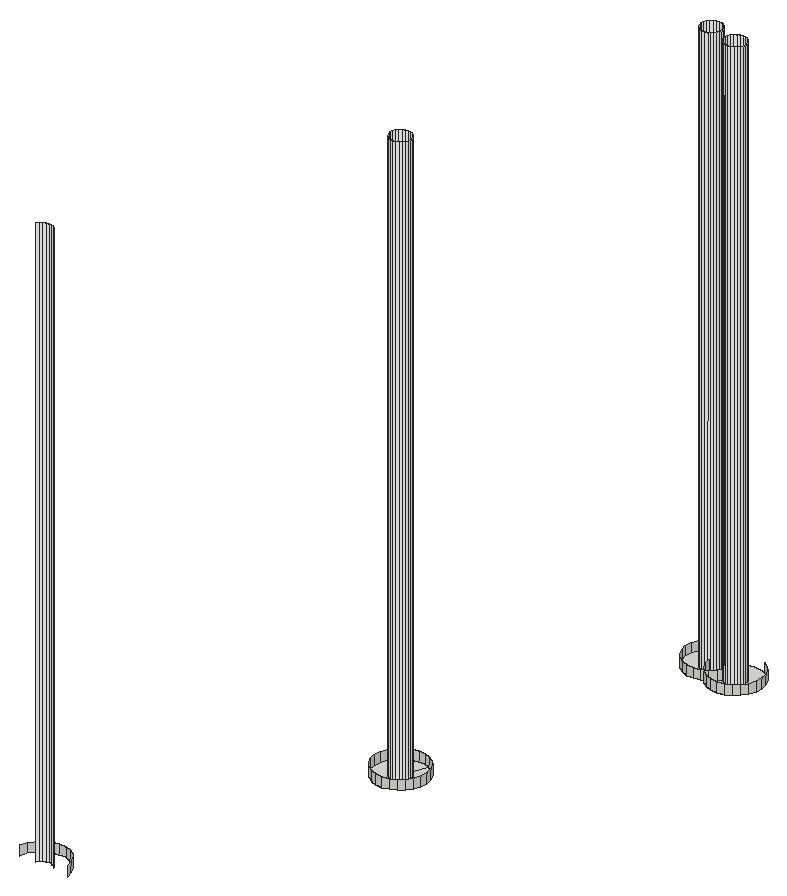
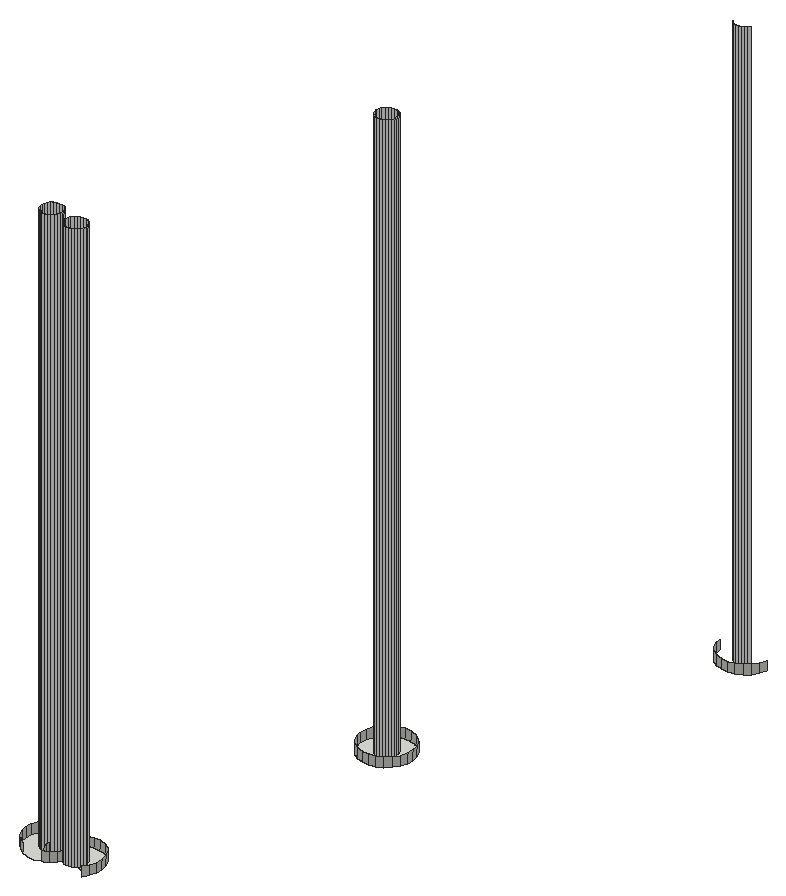
# SketchUp Ruby script. Lengths in inches.
U = 1.inch
M = Sketchup.active_model
def pt(a) = Geom::Point3d.new(a.map { |v| v * U })
def face(e, loops, mat)
  f = e.add_face(loops[0].map { |a| pt(a) })
  loops[1..].each { |l| e.add_face(l.map { |a| pt(a) }).erase! }
  f.material = f.back_material = mat if mat
  f
end
# faces: each face lists its corners as indices into pts; further lists are holes
def faces(e, pts, list, mat = nil) = list.each { |f| face(e, (f[0].is_a?(Array) ? f : [f]).map { |l| l.map { |i| pts[i] } }, mat) }
# xy, xz, yz: faces in a plane at the given z, y or x. An outline is a flat list of corners, or four numbers for a rectangle; further outlines are holes
def ring(l) = l.size == 4 ? [[l[0], l[1]], [l[2], l[1]], [l[2], l[3]], [l[0], l[3]]] : l.each_slice(2).to_a
def flat(e, list, mat, &to3) = list.each { |f| face(e, (f[0].is_a?(Array) ? f : [f]).map { |l| ring(l).map { |u, v| to3.(u, v) } }, mat) }
def xy(e, z, list, mat = nil) = flat(e, list, mat) { |x, y| [x, y, z] }
def xz(e, y, list, mat = nil) = flat(e, list, mat) { |x, z| [x, y, z] }
def yz(e, x, list, mat = nil) = flat(e, list, mat) { |y, z| [x, y, z] }
def lines(e, pts, list) = list.each { |a, b| e.add_line(pt(pts[a]), pt(pts[b])) }
# prism: a flat outline (further loops are holes) pulled along v
def prism(e, loops, v, mat = nil)
  f = face(e, loops, mat); d = Geom::Vector3d.new(v.map { |x| x * U })
  f.pushpull(f.normal.samedirection?(d) ? d.length : -d.length)
end
def box(e, o, s, mat = nil) = prism(e, [[o, [o[0] + s[0], o[1], o[2]], [o[0] + s[0], o[1] + s[1], o[2]], [o[0], o[1] + s[1], o[2]]]], [0, 0, s[2]], mat)
def at(x, y, z, deg = 0) = Geom::Transformation.translation(pt([x, y, z])) * Geom::Transformation.rotation(ORIGIN, Z_AXIS, deg.degrees)
def axes(o, x, y, z) = Geom::Transformation.new([*x, 0, *y, 0, *z, 0, *pt(o).to_a, 1])
def part(name) = M.definitions.add(name)
# library, detail: a bought-in or finely detailed component or shape, given as its bounding box
def library(name, o, s) = part(name).tap { |d| box(d.entities, o, s) }
def detail(e, o, s) = box(e.add_group.entities, o, s)
def put(e, d, t, mat = nil) = e.add_instance(d, t).tap { |i| i.material = mat if mat }
def group(e, t, mat = nil) = e.add_group.tap { |g| g.transformation = t; g.material = mat if mat }.entities
root = M.entities
M.materials.add("[Color_000]").color = [255, 255, 255]
xy(root,321.27,[[[1017.08,993.36,1017.48,993.45,1017.85,993.63,1018.16,993.9,1018.38,994.25,1018.51,994.64,1018.54,995.05,1018.45,995.45,1018.27,995.82,1018,996.125,1017.65,996.35,1017.26,996.48,1016.85,996.51,1016.45,996.42,1016.08,996.24,1015.78,995.97,1015.55,995.625,1015.42,995.23,1015.4,994.82,1015.48,994.42,1015.66,994.05,1015.94,993.75,1016.28,993.52,1016.67,993.39],[1017.01,994.31,1016.85,994.32,1016.72,994.36,1016.69,994.37,1016.55,994.46,1016.44,994.58,1016.37,994.73,1016.34,994.89,1016.35,995.05,1016.4,995.21,1016.49,995.35,1016.61,995.46,1016.76,995.53,1016.92,995.5625,1017.09,995.55,1017.22,995.51,1017.24,995.5,1017.38,995.41,1017.49,995.29,1017.5625,995.14,1017.59,994.98,1017.58,994.82,1017.53,994.66,1017.44,994.52,1017.32,994.41,1017.17,994.34]],[1016.34,993.5,1016.72,994.36,1016.69,994.37,1016.55,994.46,1016.44,994.58,1016.37,994.73,1016.34,994.89,1016.35,995.05,1016.4,995.21,1016.49,995.35,1016.61,995.46,1016.76,995.53,1016.92,995.5625,1017.09,995.55,1017.22,995.51,1017.59,996.37,1017.26,996.48,1016.85,996.51,1016.45,996.42,1016.08,996.24,1015.78,995.97,1015.55,995.625,1015.42,995.23,1015.4,994.82,1015.48,994.42,1015.66,994.05,1015.94,993.75,1016.28,993.52],[1016.72,994.36,1017.22,995.51,1017.09,995.55,1016.92,995.5625,1016.76,995.53,1016.61,995.46,1016.49,995.35,1016.4,995.21,1016.35,995.05,1016.34,994.89,1016.37,994.73,1016.44,994.58,1016.55,994.46,1016.69,994.37],[1023.97,1011.07,1024.01,1011.19,1024.04,1011.46,1024.04,1011.55,1024.03,1011.65,1024.02,1011.74,1024,1011.83,1023.97,1011.91,1023.94,1012,1023.93,1012.02,1023.92,1012.02,1023.76,1012.03,1023.6,1012.08,1023.47,1012.17,1023.4,1012.24,1023.36,1012.29,1023.28,1012.4375,1023.25,1012.6,1023.26,1012.74,1022.92,1012.9,1022.6875,1013.01,1022.68,1012.92,1022.63,1012.77,1022.54,1012.63,1022.42,1012.52,1022.32,1012.47,1022.27,1012.45,1022.11,1012.41,1021.94,1012.42,1021.79,1012.47,1021.65,1012.56,1021.54,1012.6875,1021.47,1012.83,1021.43,1013,1021.44,1013.16,1021.5,1013.32,1021.59,1013.45,1021.61,1013.47,1020.73,1013.86,1020.65,1013.73,1020.52,1013.34,1020.49,1012.93,1020.57,1012.53,1020.76,1012.16,1021.03,1011.85,1021.375,1011.625,1021.77,1011.49,1022.18,1011.47,1022.58,1011.55,1022.7,1011.62,1022.85,1011.45,1023.19,1011.23,1023.58,1011.1],[[1023.97,1011.07,1023.99,1011.07,1024.39,1011.16,1024.76,1011.34,1025.07,1011.61,1025.3,1011.96,1025.43,1012.35,1025.45,1012.76,1025.37,1013.16,1025.18,1013.53,1024.91,1013.83,1024.57,1014.0625,1024.18,1014.19,1023.77,1014.21,1023.36,1014.13,1023,1013.95,1022.6875,1013.67,1022.54,1013.45,1022.46,1013.33,1022.4,1013.13,1022.6875,1013.01,1022.68,1012.92,1022.63,1012.77,1022.54,1012.63,1022.42,1012.52,1022.32,1012.47,1022.39,1012.13,1022.57,1011.76,1022.7,1011.62,1022.85,1011.45,1023.19,1011.23,1023.58,1011.1],[1023.92,1012.02,1023.76,1012.03,1023.6,1012.08,1023.47,1012.17,1023.4,1012.24,1023.36,1012.29,1023.28,1012.4375,1023.25,1012.6,1023.26,1012.74,1023.26,1012.76,1023.3125,1012.92,1023.4,1013.06,1023.53,1013.17,1023.62,1013.21,1023.67,1013.24,1023.83,1013.27,1024,1013.26,1024.15,1013.21,1024.29,1013.12,1024.4,1013,1024.47,1012.85,1024.51,1012.6875,1024.5,1012.52,1024.45,1012.37,1024.35,1012.23,1024.23,1012.12,1024.08,1012.05,1023.93,1012.02]],
  [1023.92,1012.02,1023.93,1012.02,1023.9,1012.09,1023.86,1012.17,1023.81,1012.25,1023.71,1012.39,1023.64,1012.46,1023.58,1012.53,1023.55,1012.55,1023.48,1012.35,1023.4,1012.24,1023.47,1012.17,1023.6,1012.08,1023.76,1012.03],[1023.4,1012.24,1023.36,1012.29,1023.28,1012.4375,1023.25,1012.6,1023.26,1012.74,1023.36,1012.69,1023.44,1012.64,1023.51,1012.58,1023.55,1012.55,1023.48,1012.35],[1022.11,1012.41,1022.27,1012.45,1022.32,1012.47,1022.31,1012.53,1022.33,1012.94,1022.4,1013.13,1021.61,1013.47,1021.59,1013.45,1021.5,1013.32,1021.44,1013.16,1021.43,1013,1021.47,1012.83,1021.54,1012.6875,1021.65,1012.56,1021.79,1012.47,1021.94,1012.42],[1022.32,1012.47,1022.42,1012.52,1022.54,1012.63,1022.63,1012.77,1022.68,1012.92,1022.6875,1013.01,1022.4,1013.13,1022.33,1012.94,1022.31,1012.53]])
xy(root,321.27,[[1017.01,994.31,1017.17,994.34,1017.32,994.41,1017.44,994.52,1017.53,994.66,1017.58,994.82,1017.59,994.98,1017.5625,995.14,1017.49,995.29,1017.38,995.41,1017.24,995.5,1017.22,995.51,1016.72,994.36,1016.85,994.32],[1023.93,1012.02,1024.08,1012.05,1024.23,1012.12,1024.35,1012.23,1024.45,1012.37,1024.5,1012.52,1024.51,1012.6875,1024.47,1012.85,1024.4,1013,1024.29,1013.12,1024.15,1013.21,1024,1013.26,1023.83,1013.27,1023.67,1013.24,1023.62,1013.21,1023.63,1013.15,1023.61,1012.74,1023.55,1012.55,1023.58,1012.53,1023.64,1012.46,1023.71,1012.39,1023.81,1012.25,1023.86,1012.17,1023.9,1012.09],[1023.55,1012.55,1023.51,1012.58,1023.44,1012.64,1023.36,1012.69,1023.26,1012.74,1023.26,1012.76,1023.3125,1012.92,1023.4,1013.06,1023.53,1013.17,1023.62,1013.21,1023.63,1013.15,1023.61,1012.74],[1022.6875,1013.01,1022.4,1013.13,1021.61,1013.47,1021.71,1013.5625,1021.86,1013.64,1022.02,1013.67,1022.18,1013.66,1022.34,1013.61,1022.48,1013.52,1022.54,1013.45,1022.58,1013.39,1022.66,1013.25,1022.69,1013.09]],"[Color_000]")
p = [[1010.57,976.74,321.27],[1010.48,977.15,321.27],[1010.48,977.15,321.86],[1010.57,976.74,321.86],[1007.58,977.32,321.27],[1007.45,976.93,321.27],
  [1007.45,976.93,321.86],[1007.58,977.32,321.86],[1008.52,977.04,321.27],[1008.43,976.91,321.27],[1008.43,976.91,357.27],[1008.52,977.04,357.27],
  [1008.64,977.15,321.27],[1008.64,977.15,357.27],[1009.52,976.98,321.27],[1009.41,977.11,321.27],[1009.41,977.11,357.27],[1009.52,976.98,357.27],
  [1009.27,977.2,321.27],[1009.27,977.2,357.27],[1010.3,977.51,321.27],[1010.3,977.51,321.86],[1008.79,977.23,321.27],[1008.79,977.23,357.27],
  [1008.95,977.26,321.27],[1008.95,977.26,357.27],[1009.11,977.25,321.27],[1009.11,977.25,357.27],[1009.24,977.21,321.27],[1007.8,977.66,321.27],
  [1007.8,977.66,321.86],[1010.03,977.82,321.27],[1010.03,977.82,321.86],[1008.11,977.93,321.27],[1008.11,977.93,321.86],[1009.68,978.05,321.27],
  [1009.68,978.05,321.86],[1008.48,978.12,321.27],[1008.48,978.12,321.86],[1009.62,978.07,321.27],[1009.29,978.18,321.27],[1009.29,978.18,321.86],
  [1008.88,978.2,321.27],[1008.88,978.2,321.86],[1016.28,993.52,321.27],[1016.34,993.5,321.27],[1016.67,993.39,321.27],[1016.67,993.39,321.86],
  [1016.28,993.52,321.86],[1017.08,993.36,321.27],[1017.08,993.36,321.86],[1017.48,993.45,321.27],[1017.48,993.45,321.86],[1017.85,993.63,321.27],
  [1017.85,993.63,321.86],[1015.94,993.75,321.27],[1015.94,993.75,321.86],[1018.16,993.9,321.27],[1018.16,993.9,321.86],[1015.66,994.05,321.27],
  [1015.66,994.05,321.86],[1018.38,994.25,321.27],[1018.38,994.25,321.86],[1015.48,994.42,321.27],[1015.48,994.42,321.86],[1018.51,994.64,321.27],
  [1018.51,994.64,321.86],[1016.69,994.37,321.27],[1016.72,994.36,321.27],[1016.85,994.32,321.27],[1016.85,994.32,357.27],[1016.69,994.37,357.27],
  [1017.01,994.31,321.27],[1017.01,994.31,357.27],[1017.17,994.34,321.27],[1017.17,994.34,357.27],[1017.32,994.41,321.27],[1017.32,994.41,357.27],
  [1015.4,994.82,321.27],[1015.4,994.82,321.86],[1016.55,994.46,321.27],[1016.55,994.46,357.27],[1017.44,994.52,321.27],[1017.44,994.52,357.27],
  [1016.44,994.58,321.27],[1016.44,994.58,357.27],[1017.53,994.66,321.27],[1017.53,994.66,357.27],[1016.37,994.73,321.27],[1016.37,994.73,357.27],
  [1018.54,995.05,321.27],[1018.54,995.05,321.86],[1016.34,994.89,321.27],[1016.34,994.89,357.27],[1017.58,994.82,321.27],[1017.58,994.82,357.27],
  [1015.42,995.23,321.27],[1015.42,995.23,321.86],[1017.59,994.98,321.27],[1017.59,994.98,357.27],[1016.35,995.05,321.27],[1016.35,995.05,357.27],
  [1017.5625,995.14,321.27],[1017.5625,995.14,357.27],[1018.45,995.45,321.27],[1018.45,995.45,321.86],[1016.4,995.21,321.27],[1016.4,995.21,357.27],
  [1017.49,995.29,321.27],[1017.49,995.29,357.27],[1015.55,995.625,321.27],[1015.55,995.625,321.86],[1016.49,995.35,321.27],[1016.49,995.35,357.27],
  [1016.61,995.46,321.27],[1016.61,995.46,357.27],[1017.38,995.41,321.27],[1017.38,995.41,357.27],[1017.24,995.5,321.27],[1017.24,995.5,357.27],
  [1016.76,995.53,321.27],[1016.76,995.53,357.27],[1016.92,995.5625,321.27],[1016.92,995.5625,357.27],[1017.22,995.51,321.27],[1017.09,995.55,321.27],
  [1017.09,995.55,357.27],[1018.27,995.82,321.27],[1018.27,995.82,321.86],[1015.78,995.97,321.27],[1015.78,995.97,321.86],[1018,996.125,321.27],
  [1018,996.125,321.86],[1016.08,996.24,321.27],[1016.08,996.24,321.86],[1017.65,996.35,321.27],[1017.65,996.35,321.86],[1016.45,996.42,321.27],
  [1016.45,996.42,321.86],[1016.85,996.51,321.27],[1016.85,996.51,321.86],[1017.59,996.37,321.27],[1017.26,996.48,321.27],[1017.26,996.48,321.86],
  [1023.19,1011.23,321.27],[1023.58,1011.1,321.27],[1023.58,1011.1,321.86],[1023.19,1011.23,321.86],[1023.97,1011.07,321.27],[1023.99,1011.07,321.27],
  [1023.99,1011.07,321.86],[1024.39,1011.16,321.27],[1024.39,1011.16,321.86],[1022.85,1011.45,321.27],[1022.85,1011.45,321.86],[1024.76,1011.34,321.27],
  [1024.76,1011.34,321.86],[1025.07,1011.61,321.27],[1025.07,1011.61,321.86],[1021.375,1011.625,321.27],[1021.77,1011.49,321.27],[1021.77,1011.49,321.86],
  [1021.375,1011.625,321.86],[1022.18,1011.47,321.27],[1022.18,1011.47,321.86],[1022.58,1011.55,321.27],[1022.58,1011.55,321.86],[1022.57,1011.76,321.27],
  [1022.7,1011.62,321.27],[1022.7,1011.62,321.86],[1022.57,1011.76,321.86],[1021.03,1011.85,321.27],[1021.03,1011.85,321.86],[1022.95,1011.74,321.27],
  [1022.95,1011.74,321.86],[1025.3,1011.96,321.27],[1025.3,1011.96,321.86],[1023.25,1012.01,321.27],[1023.25,1012.01,321.86],[1022.39,1012.13,321.27],
  [1022.39,1012.13,321.86],[1020.76,1012.16,321.27],[1020.76,1012.16,321.86],[1023.4,1012.24,321.27],[1023.48,1012.35,321.27],[1023.48,1012.35,321.86],
  [1023.6,1012.08,321.27],[1023.76,1012.03,321.27],[1023.76,1012.03,357.27],[1023.6,1012.08,357.27],[1023.92,1012.02,321.27],[1023.92,1012.02,357.27],
  [1023.93,1012.02,321.27],[1024.08,1012.05,321.27],[1024.08,1012.05,357.27],[1024.23,1012.12,321.27],[1024.23,1012.12,357.27],[1025.43,1012.35,321.27],
  [1025.43,1012.35,321.86],[1022.31,1012.53,321.27],[1022.32,1012.47,321.27],[1022.31,1012.53,321.86],[1023.47,1012.17,321.27],[1023.47,1012.17,357.27],
  [1024.35,1012.23,321.27],[1024.35,1012.23,357.27],[1020.57,1012.53,321.27],[1020.57,1012.53,321.86],[1023.36,1012.29,321.27],[1023.36,1012.29,357.27],
  [1024.45,1012.37,321.27],[1024.45,1012.37,357.27],[1023.28,1012.4375,321.27],[1023.28,1012.4375,357.27],[1025.45,1012.76,321.27],[1025.45,1012.76,321.86],
  [1021.79,1012.47,321.27],[1021.94,1012.42,321.27],[1021.94,1012.42,357.27],[1021.79,1012.47,357.27],[1022.11,1012.41,321.27],[1022.11,1012.41,357.27],
  [1022.27,1012.45,321.27],[1022.27,1012.45,357.27],[1022.42,1012.52,321.27],[1022.42,1012.52,357.27],[1023.25,1012.6,321.27],[1023.25,1012.6,357.27],
  [1023.25,1012.6,353.41],[1023.25,1012.6,351.28],[1023.25,1012.6,335.125],[1023.25,1012.6,333],[1023.55,1012.55,321.27],[1023.61,1012.74,321.27],
  [1023.61,1012.74,321.86],[1024.5,1012.52,321.27],[1024.5,1012.52,357.27],[1020.49,1012.93,321.27],[1020.49,1012.93,321.86],[1021.65,1012.56,321.27],
  [1021.65,1012.56,357.27],[1022.33,1012.94,321.27],[1022.33,1012.94,321.86],[1022.54,1012.63,321.27],[1022.54,1012.63,357.27],[1024.51,1012.6875,321.27],
  [1024.51,1012.6875,357.27],[1021.54,1012.6875,321.27],[1021.54,1012.6875,357.27],[1022.63,1012.77,321.27],[1022.63,1012.77,357.27],[1023.26,1012.76,321.27],
  [1023.26,1012.74,321.27],[1023.26,1012.76,357.27],[1021.47,1012.83,321.27],[1021.47,1012.83,357.27],[1023.63,1013.15,321.27],[1023.63,1013.15,321.86],
  [1024.47,1012.85,321.27],[1024.47,1012.85,357.27],[1021.43,1013,321.27],[1021.43,1013,357.27],[1022.68,1012.92,321.27],[1022.68,1012.92,357.27],
  [1023.3125,1012.92,321.27],[1023.3125,1012.92,357.27],[1025.37,1013.16,321.27],[1025.37,1013.16,321.86],[1020.52,1013.34,321.27],[1020.52,1013.34,321.86],
  [1022.46,1013.33,321.27],[1022.4,1013.13,321.27],[1022.46,1013.33,321.86],[1022.6875,1013.01,321.27],[1022.69,1013.09,321.27],[1022.69,1013.09,357.27],
  [1023.4,1013.06,321.27],[1023.4,1013.06,357.27],[1024.4,1013,321.27],[1024.4,1013,357.27],[1021.44,1013.16,321.27],[1021.44,1013.16,357.27],
  [1024.29,1013.12,321.27],[1024.29,1013.12,357.27],[1022.66,1013.25,321.27],[1022.66,1013.25,357.27],[1023.53,1013.17,321.27],[1023.53,1013.17,357.27],
  [1024.15,1013.21,321.27],[1024.15,1013.21,357.27],[1021.5,1013.32,321.27],[1021.5,1013.32,357.27],[1022.58,1013.39,321.27],[1022.58,1013.39,357.27],
  [1023.67,1013.24,321.27],[1023.62,1013.21,321.27],[1023.67,1013.24,357.27],[1023.55,1013.56,321.27],[1023.55,1013.56,321.86],[1023.83,1013.27,321.27],
  [1023.83,1013.27,357.27],[1024,1013.26,321.27],[1024,1013.26,357.27],[1025.18,1013.53,321.27],[1025.18,1013.53,321.86],[1020.65,1013.73,321.27],
  [1020.65,1013.73,321.86],[1021.59,1013.45,321.27],[1021.59,1013.45,357.27],[1022.6875,1013.67,321.27],[1022.54,1013.45,321.27],[1022.6875,1013.67,321.86],
  [1022.48,1013.52,321.27],[1022.48,1013.52,357.27],[1021.71,1013.5625,321.27],[1021.61,1013.47,321.27],[1021.71,1013.5625,357.27],[1022.34,1013.61,321.27],
  [1022.34,1013.61,357.27],[1024.91,1013.83,321.27],[1024.91,1013.83,321.86],[1021.86,1013.64,321.27],[1021.86,1013.64,357.27],[1022.02,1013.67,321.27],
  [1022.02,1013.67,357.27],[1022.18,1013.66,321.27],[1022.18,1013.66,357.27],[1023.37,1013.92,321.27],[1023.37,1013.92,321.86],[1020.87,1014.07,321.27],
  [1020.73,1013.86,321.27],[1020.87,1014.07,321.86],[1023,1013.95,321.27],[1023,1013.95,321.86],[1024.57,1014.0625,321.27],[1024.57,1014.0625,321.86],
  [1023.36,1014.13,321.27],[1023.24,1014.07,321.27],[1023.24,1014.07,321.86],[1023.36,1014.13,321.86]]
faces(root,p,[[0,1,2,3],[4,5,6,7],[1,20,21,2],[29,4,7,30],[20,31,32,21],[33,29,30,34],[31,35,36,32],[37,33,34,38],
  [35,39,40,41,36],[42,37,38,43],[40,42,43,41],[44,45,46,47,48],[46,49,50,47],[49,51,52,50],[51,53,54,52],[55,44,48,56],
  [53,57,58,54],[59,55,56,60],[57,61,62,58],[63,59,60,64],[61,65,66,62],[78,63,64,79],[65,90,91,66],[96,78,79,97],
  [90,104,105,91],[110,96,97,111],[104,127,128,105],[129,110,111,130],[127,131,132,128],[133,129,130,134],[131,135,136,132],[137,133,134,138],
  [139,137,138,140],[135,141,142,143,136],[142,139,140,143],[144,145,146,147],[145,148,149,150,146],[149,151,152,150],[153,144,147,154],[151,155,156,152],
  [155,157,158,156],[159,160,161,162],[160,163,164,161],[163,165,166,164],[167,168,153,154,169,170],[171,159,162,172],[165,168,173,174,169,166],[157,175,176,158],
  [173,177,178,174],[179,167,170,180],[181,171,172,182],[177,183,184,185,178],[175,197,198,176],[199,200,179,180,201],[206,181,182,207],[197,214,215,198],
  [184,232,233,234,185],[237,206,207,238],[241,199,201,242],[233,256,257,234],[214,266,267,215],[268,237,238,269],[270,271,241,242,272],[256,295,297,298,257],
  [266,303,304,267],[305,268,269,306],[309,310,270,272,311],[303,319,320,304],[297,327,328,298],[329,330,305,306,331],[332,309,311,333],[319,334,335,320],
  [336,337,332,333,338,339]])
faces(root,p,[[8,9,10,11],[12,8,11,13],[14,15,16,17],[15,18,19,16],[22,12,13,23],[24,22,23,25],[26,24,25,27],[18,28,26,27,19],
  [67,68,69,70,71],[69,72,73,70],[72,74,75,73],[74,76,77,75],[80,67,71,81],[76,82,83,77],[84,80,81,85],[82,86,87,83],
  [88,84,85,89],[92,88,89,93],[86,94,95,87],[94,98,99,95],[100,92,93,101],[98,102,103,99],[106,100,101,107],[102,108,109,103],
  [112,106,107,113],[114,112,113,115],[108,116,117,109],[116,118,119,117],[120,114,115,121],[122,120,121,123],[118,124,125,126,119],[125,122,123,126],
  [186,187,188,189],[187,190,191,188],[190,192,193,194,191],[193,195,196,194],[202,186,189,203],[195,204,205,196],[208,183,202,203,209],[204,210,211,205],
  [212,208,209,213],[216,217,218,219],[217,220,221,218],[220,222,223,221],[222,200,224,225,223],[226,212,213,227,228,229,230,231],[210,235,236,211],[239,216,219,240],
  [224,243,244,225],[235,245,246,236],[247,239,240,248],[243,249,250,244],[251,252,226,231,230,229,228,227,253],[254,247,248,255],[245,258,259,246],[260,254,255,261],
  [249,262,263,250],[264,251,253,265],[262,273,274,275,263],[276,264,265,277],[258,278,279,259],[280,260,261,281],[278,282,283,279],[274,284,285,275],
  [286,276,277,287],[282,288,289,283],[290,280,281,291],[284,292,293,285],[294,295,286,287,296],[299,294,296,300],[288,301,302,289],[307,290,291,308],
  [301,299,300,302],[292,310,312,313,293],[314,315,307,308,316],[312,317,318,313],[321,314,316,322],[323,321,322,324],[317,325,326,318],[325,323,324,326]],"[Color_000]")
